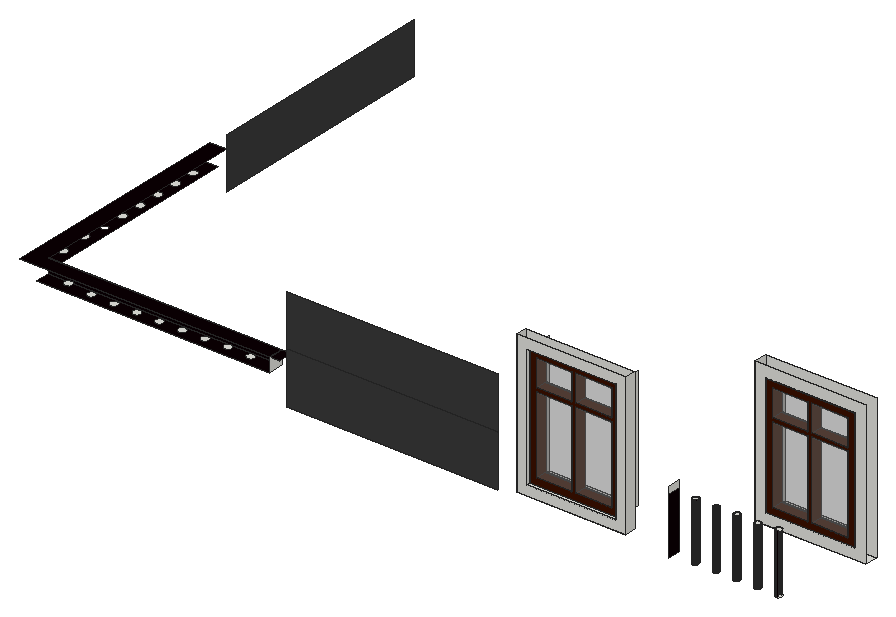
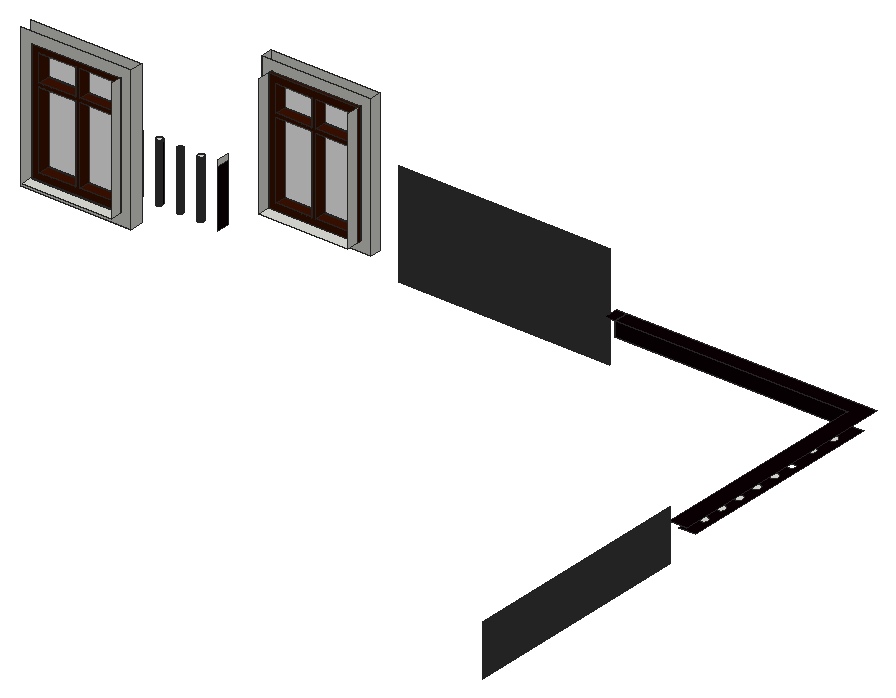
# SketchUp Ruby script. Lengths in inches.
U = 1.inch
M = Sketchup.active_model
def pt(a) = Geom::Point3d.new(a.map { |v| v * U })
def face(e, loops, mat)
  f = e.add_face(loops[0].map { |a| pt(a) })
  loops[1..].each { |l| e.add_face(l.map { |a| pt(a) }).erase! }
  f.material = f.back_material = mat if mat
  f
end
# faces: each face lists its corners as indices into pts; further lists are holes
def faces(e, pts, list, mat = nil) = list.each { |f| face(e, (f[0].is_a?(Array) ? f : [f]).map { |l| l.map { |i| pts[i] } }, mat) }
# xy, xz, yz: faces in a plane at the given z, y or x. An outline is a flat list of corners, or four numbers for a rectangle; further outlines are holes
def ring(l) = l.size == 4 ? [[l[0], l[1]], [l[2], l[1]], [l[2], l[3]], [l[0], l[3]]] : l.each_slice(2).to_a
def flat(e, list, mat, &to3) = list.each { |f| face(e, (f[0].is_a?(Array) ? f : [f]).map { |l| ring(l).map { |u, v| to3.(u, v) } }, mat) }
def xy(e, z, list, mat = nil) = flat(e, list, mat) { |x, y| [x, y, z] }
def xz(e, y, list, mat = nil) = flat(e, list, mat) { |x, z| [x, y, z] }
def yz(e, x, list, mat = nil) = flat(e, list, mat) { |y, z| [x, y, z] }
def lines(e, pts, list) = list.each { |a, b| e.add_line(pt(pts[a]), pt(pts[b])) }
# prism: a flat outline (further loops are holes) pulled along v
def prism(e, loops, v, mat = nil)
  f = face(e, loops, mat); d = Geom::Vector3d.new(v.map { |x| x * U })
  f.pushpull(f.normal.samedirection?(d) ? d.length : -d.length)
end
def box(e, o, s, mat = nil) = prism(e, [[o, [o[0] + s[0], o[1], o[2]], [o[0] + s[0], o[1] + s[1], o[2]], [o[0], o[1] + s[1], o[2]]]], [0, 0, s[2]], mat)
def at(x, y, z, deg = 0) = Geom::Transformation.translation(pt([x, y, z])) * Geom::Transformation.rotation(ORIGIN, Z_AXIS, deg.degrees)
def axes(o, x, y, z) = Geom::Transformation.new([*x, 0, *y, 0, *z, 0, *pt(o).to_a, 1])
def part(name) = M.definitions.add(name)
# library, detail: a bought-in or finely detailed component or shape, given as its bounding box
def library(name, o, s) = part(name).tap { |d| box(d.entities, o, s) }
def detail(e, o, s) = box(e.add_group.entities, o, s)
def put(e, d, t, mat = nil) = e.add_instance(d, t).tap { |i| i.material = mat if mat }
def group(e, t, mat = nil) = e.add_group.tap { |g| g.transformation = t; g.material = mat if mat }.entities
root = M.entities
M.materials.add("[Color C08]").color = [60, 17, 0]
M.materials.add("[Color M07]").color = [58, 58, 58]
M.materials.add("[Metal Seamed]").color = [11, 0, 4]
M.materials.add("[Translucent Glass Gray]").color = [128, 128, 128]
M.materials["[Translucent Glass Gray]"].alpha = 0.5
c1 = part("Group\#3")
xy(c1.entities,0,[[0,0,51.6875,4]],"[Color C08]")
xy(c1.entities,4.05,[[4.05,0,24.41,4],[24.41,0,26.55,4],[26.55,0,47.64,4]],"[Color C08]")
xy(c1.entities,49.59,[[4.05,0,24.41,4],[26.55,0,47.64,4]],"[Color C08]")
xy(c1.entities,51.6875,[[4.05,0,24.41,4],[26.55,0,47.64,4]],"[Color C08]")
xy(c1.entities,67.57,[[4.05,0,24.41,4],[26.55,0,47.64,4]],"[Color C08]")
xy(c1.entities,71.625,[[0,0,51.6875,4]],"[Color C08]")
xz(c1.entities,0,[[[0,0,51.6875,71.625],[4.05,4.05,4.05,49.59,24.41,49.59,24.41,4.05,26.55,4.05,26.55,49.59,47.64,49.59,47.64,4.05],[26.55,51.6875,47.64,67.57],[4.05,51.6875,24.41,67.57]]],"[Color C08]")
xz(c1.entities,0,[[4.05,4.05,24.41,49.59],[26.55,4.05,47.64,49.59],[4.05,51.6875,24.41,67.57],[26.55,51.6875,47.64,67.57]],"[Translucent Glass Gray]")
xz(c1.entities,4,[[[0,0,51.6875,71.625],[4.05,4.05,4.05,49.59,24.41,49.59,24.41,4.05,26.55,4.05,26.55,49.59,47.64,49.59,47.64,4.05],[26.55,51.6875,47.64,67.57],[4.05,51.6875,24.41,67.57]]],"[Color C08]")
yz(c1.entities,0,[[0,0,4,71.625]],"[Color C08]")
yz(c1.entities,4.05,[[0,4.05,4,49.59],[0,51.6875,4,67.57]],"[Color C08]")
yz(c1.entities,24.41,[[0,4.05,4,49.59],[0,51.6875,4,67.57]],"[Color C08]")
yz(c1.entities,26.55,[[0,4.05,4,49.59],[0,51.6875,4,67.57]],"[Color C08]")
yz(c1.entities,47.64,[[0,4.05,4,49.59],[0,51.6875,4,67.57]],"[Color C08]")
yz(c1.entities,51.6875,[[0,0,4,71.625]],"[Color C08]")
xy(root,156,[[381.34,72.62,380.91,72.67,380.5,72.83,380.14,73.09,379.86,73.43,379.6875,73.83,379.62,74.27,379.67,74.71,379.83,75.12,380.09,75.47,380.43,75.75,380.84,75.93,381.27,75.99,381.71,75.94,382.12,75.78,382.48,75.52,382.75,75.18,382.93,74.78,382.99,74.34,382.95,73.9,382.79,73.49,382.53,73.14,382.18,72.86,381.78,72.68],[392.97,72.62,392.53,72.67,392.12,72.83,391.76,73.09,391.49,73.43,391.3125,73.83,391.25,74.27,391.29,74.71,391.45,75.12,391.71,75.47,392.06,75.75,392.46,75.93,392.9,75.99,393.33,75.94,393.75,75.78,394.1,75.52,394.375,75.18,394.55,74.78,394.62,74.34,394.57,73.9,394.41,73.49,394.15,73.14,393.81,72.86,393.4,72.68],[404.59,72.62,404.16,72.67,403.75,72.83,403.39,73.09,403.11,73.43,402.9375,73.83,402.87,74.27,402.92,74.71,403.08,75.12,403.34,75.47,403.68,75.75,404.09,75.93,404.52,75.99,404.96,75.94,405.37,75.78,405.73,75.52,406,75.18,406.18,74.78,406.24,74.34,406.2,73.9,406.04,73.49,405.78,73.14,405.43,72.86,405.03,72.68],[416.22,72.62,415.78,72.67,415.37,72.83,415.01,73.09,414.74,73.43,414.5625,73.83,414.5,74.27,414.54,74.71,414.7,75.12,414.96,75.47,415.31,75.75,415.71,75.93,416.15,75.99,416.58,75.94,417,75.78,417.35,75.52,417.625,75.18,417.8,74.78,417.87,74.34,417.82,73.9,417.66,73.49,417.4,73.14,417.06,72.86,416.65,72.68],[427.84,72.62,427.41,72.67,427,72.83,426.64,73.09,426.36,73.43,426.1875,73.83,426.12,74.27,426.17,74.71,426.33,75.12,426.59,75.47,426.93,75.75,427.34,75.93,427.77,75.99,428.21,75.94,428.62,75.78,428.98,75.52,429.25,75.18,429.43,74.78,429.49,74.34,429.45,73.9,429.29,73.49,429.03,73.14,428.68,72.86,428.28,72.68]])
xy(root,165.94,[[388.97,106.41,451.12,113.66]])
xy(root,166.3,[[291.9,60.85,353.07,67.28]])
xy(root,171.85,[[297.45,60.85,347.52,67.28],[297.45,67.28,347.52,76.28]])
xy(root,171.98,[[395.02,106.41,445.08,113.66],[395.02,113.66,445.08,119.66]])
xy(root,176.54,[[21.75,62.41,152.3,70.73]],"[Metal Seamed]")
xy(root,177,[[61.41,65.07,61.9,65.2,62.34,65.44,62.71,65.79,62.97,66.23,63.11,66.71,63.11,67.22,62.99,67.71,62.75,68.15,62.39,68.52,61.96,68.78,61.47,68.91,60.97,68.92,60.48,68.8,60.03,68.55,59.67,68.2,59.41,67.77,59.27,67.28,59.26,66.78,59.39,66.29,59.63,65.84,59.98,65.48,60.42,65.22,60.9,65.08]])
xy(root,177.0625,[[86.91,65.07,87.4,65.2,87.84,65.44,88.21,65.79,88.47,66.23,88.61,66.71,88.61,67.22,88.49,67.71,88.25,68.15,87.89,68.52,87.46,68.78,86.97,68.91,86.47,68.92,85.98,68.8,85.53,68.55,85.17,68.2,84.91,67.77,84.77,67.28,84.76,66.78,84.89,66.29,85.13,65.84,85.48,65.48,85.92,65.22,86.4,65.08]])
xy(root,177.125,[[74.16,65.07,74.65,65.2,75.09,65.44,75.46,65.79,75.72,66.23,75.86,66.71,75.86,67.22,75.74,67.71,75.5,68.15,75.14,68.52,74.71,68.78,74.22,68.91,73.72,68.92,73.23,68.8,72.78,68.55,72.42,68.2,72.16,67.77,72.02,67.28,72.01,66.78,72.14,66.29,72.38,65.84,72.73,65.48,73.17,65.22,73.65,65.08]])
xy(root,177.1875,[[48.66,65.07,49.15,65.2,49.59,65.44,49.96,65.79,50.22,66.23,50.36,66.71,50.36,67.22,50.24,67.71,50,68.15,49.64,68.52,49.21,68.78,48.72,68.91,48.22,68.92,47.73,68.8,47.28,68.55,46.92,68.2,46.66,67.77,46.52,67.28,46.51,66.78,46.64,66.29,46.88,65.84,47.23,65.48,47.67,65.22,48.15,65.08],[99.66,65.07,100.15,65.2,100.59,65.44,100.96,65.79,101.22,66.23,101.36,66.71,101.36,67.22,101.24,67.71,101,68.15,100.64,68.52,100.21,68.78,99.72,68.91,99.22,68.92,98.73,68.8,98.28,68.55,97.92,68.2,97.66,67.77,97.52,67.28,97.51,66.78,97.64,66.29,97.88,65.84,98.23,65.48,98.67,65.22,99.15,65.08]])
xy(root,177.3125,[[112.41,65.07,112.9,65.2,113.34,65.44,113.71,65.79,113.97,66.23,114.11,66.71,114.11,67.22,113.99,67.71,113.75,68.15,113.39,68.52,112.96,68.78,112.47,68.91,111.97,68.92,111.48,68.8,111.03,68.55,110.67,68.2,110.41,67.77,110.27,67.28,110.26,66.78,110.39,66.29,110.63,65.84,110.98,65.48,111.42,65.22,111.9,65.08]])
xy(root,177.4375,[[137.97,65.07,138.46,65.2,138.91,65.44,139.27,65.79,139.53,66.23,139.67,66.71,139.68,67.22,139.55,67.71,139.31,68.15,138.96,68.52,138.52,68.78,138.04,68.91,137.53,68.92,137.04,68.8,136.6,68.55,136.23,68.2,135.97,67.77,135.83,67.28,135.83,66.78,135.95,66.29,136.2,65.84,136.55,65.48,136.98,65.22,137.47,65.08]])
xy(root,177.75,[[125.16,65.07,125.65,65.2,126.09,65.44,126.46,65.79,126.72,66.23,126.86,66.71,126.86,67.22,126.74,67.71,126.5,68.15,126.14,68.52,125.71,68.78,125.22,68.91,124.72,68.92,124.23,68.8,123.78,68.55,123.42,68.2,123.16,67.77,123.02,67.28,123.01,66.78,123.14,66.29,123.38,65.84,123.73,65.48,124.17,65.22,124.65,65.08]])
xy(root,178.3125,[[35.91,65.07,36.4,65.2,36.84,65.44,37.21,65.79,37.47,66.23,37.61,66.71,37.61,67.22,37.49,67.71,37.25,68.15,36.89,68.52,36.46,68.78,35.97,68.91,35.47,68.92,34.98,68.8,34.53,68.55,34.17,68.2,33.91,67.77,33.77,67.28,33.76,66.78,33.89,66.29,34.13,65.84,34.48,65.48,34.92,65.22,35.4,65.08]])
xy(root,178.35,[[[12.3125,71.24,21.75,188.85],[17.07,113.4,17.62,113.43,18.15,113.6,18.62,113.9,18.99,114.31,19.24,114.8,19.36,115.35,19.33,115.9,19.17,116.43,18.87,116.89,18.45,117.27,17.96,117.52,17.42,117.64,16.87,117.61,16.34,117.44,15.87,117.14,15.5,116.73,15.24,116.24,15.125,115.7,15.15,115.14,15.32,114.62,15.62,114.15,16.03,113.78,16.52,113.52]]],"[Metal Seamed]")
xy(root,178.875,[[17.07,150.34,17.62,150.37,18.15,150.54,18.62,150.84,18.99,151.25,19.24,151.74,19.36,152.28,19.33,152.84,19.17,153.37,18.87,153.83,18.45,154.21,17.96,154.46,17.42,154.58,16.87,154.55,16.34,154.38,15.87,154.08,15.5,153.67,15.24,153.18,15.125,152.64,15.15,152.08,15.32,151.55,15.62,151.09,16.03,150.71,16.52,150.46]])
xy(root,178.9375,[[17.07,138.03,17.62,138.06,18.15,138.22,18.62,138.52,18.99,138.94,19.24,139.43,19.36,139.97,19.33,140.52,19.17,141.05,18.87,141.52,18.45,141.89,17.96,142.15,17.42,142.26,16.87,142.24,16.34,142.07,15.87,141.77,15.5,141.36,15.24,140.87,15.125,140.32,15.15,139.77,15.32,139.24,15.62,138.77,16.03,138.4,16.52,138.15],[17.07,174.97,17.62,174.99,18.15,175.16,18.62,175.46,18.99,175.87,19.24,176.37,19.36,176.91,19.33,177.46,19.17,177.99,18.87,178.46,18.45,178.83,17.96,179.08,17.42,179.2,16.87,179.18,16.34,179.01,15.87,178.71,15.5,178.3,15.24,177.8,15.125,177.26,15.15,176.71,15.32,176.18,15.62,175.71,16.03,175.34,16.52,175.08]])
xy(root,179,[[17.07,125.72,17.62,125.74,18.15,125.91,18.62,126.21,18.99,126.62,19.24,127.12,19.36,127.66,19.33,128.21,19.17,128.74,18.87,129.21,18.45,129.58,17.96,129.83,17.42,129.95,16.87,129.93,16.34,129.76,15.87,129.46,15.5,129.05,15.24,128.55,15.125,128.01,15.15,127.46,15.32,126.93,15.62,126.46,16.03,126.09,16.52,125.83]])
xy(root,179.0625,[[17.07,162.65,17.62,162.68,18.15,162.85,18.62,163.15,18.99,163.56,19.24,164.05,19.36,164.6,19.33,165.15,19.17,165.68,18.87,166.14,18.45,166.52,17.96,166.77,17.42,166.89,16.87,166.86,16.34,166.69,15.87,166.39,15.5,165.98,15.24,165.49,15.125,164.95,15.15,164.39,15.32,163.87,15.62,163.4,16.03,163.03,16.52,162.77]])
xy(root,179.5625,[[17.07,84.28,17.62,84.31,18.15,84.47,18.62,84.77,18.99,85.19,19.24,85.68,19.36,86.22,19.33,86.77,19.17,87.3,18.87,87.77,18.45,88.14,17.96,88.4,17.42,88.51,16.87,88.49,16.34,88.32,15.87,88.02,15.5,87.61,15.24,87.12,15.125,86.57,15.15,86.02,15.32,85.49,15.62,85.02,16.03,84.65,16.52,84.4]])
xy(root,180.25,[[17.07,99.09,17.62,99.12,18.15,99.29,18.62,99.59,18.99,100,19.24,100.49,19.36,101.03,19.33,101.59,19.17,102.12,18.87,102.58,18.45,102.96,17.96,103.21,17.42,103.33,16.87,103.3,16.34,103.13,15.87,102.83,15.5,102.42,15.24,101.93,15.125,101.39,15.15,100.83,15.32,100.3,15.62,99.84,16.03,99.46,16.52,99.21]])
xy(root,184.4375,[[12.3125,62.41,152.3,62.41,152.3,70.73,21.75,70.73,21.75,195.41,12.3125,195.41],[152.3,62.41,158,70.73]],"[Metal Seamed]")
xy(root,188.3125,[[416.22,72.62,416.65,72.68,417.06,72.86,417.4,73.14,417.66,73.49,417.82,73.9,417.87,74.34,417.8,74.78,417.625,75.18,417.35,75.52,417,75.78,416.58,75.94,416.15,75.99,415.71,75.93,415.31,75.75,414.96,75.47,414.7,75.12,414.54,74.71,414.5,74.27,414.5625,73.83,414.74,73.43,415.01,73.09,415.37,72.83,415.78,72.67]])
xy(root,188.4375,[[381.34,72.62,381.78,72.68,382.18,72.86,382.53,73.14,382.79,73.49,382.95,73.9,382.99,74.34,382.93,74.78,382.75,75.18,382.48,75.52,382.12,75.78,381.71,75.94,381.27,75.99,380.84,75.93,380.43,75.75,380.09,75.47,379.83,75.12,379.67,74.71,379.62,74.27,379.6875,73.83,379.86,73.43,380.14,73.09,380.5,72.83,380.91,72.67]])
xy(root,188.75,[[404.59,72.62,405.03,72.68,405.43,72.86,405.78,73.14,406.04,73.49,406.2,73.9,406.24,74.34,406.18,74.78,406,75.18,405.73,75.52,405.37,75.78,404.96,75.94,404.52,75.99,404.09,75.93,403.68,75.75,403.34,75.47,403.08,75.12,402.92,74.71,402.87,74.27,402.9375,73.83,403.11,73.43,403.39,73.09,403.75,72.83,404.16,72.67]])
xy(root,189.4375,[[427.84,72.62,428.28,72.68,428.68,72.86,429.03,73.14,429.29,73.49,429.45,73.9,429.49,74.34,429.43,74.78,429.25,75.18,428.98,75.52,428.62,75.78,428.21,75.94,427.77,75.99,427.34,75.93,426.93,75.75,426.59,75.47,426.33,75.12,426.17,74.71,426.12,74.27,426.1875,73.83,426.36,73.43,426.64,73.09,427,72.83,427.41,72.67]])
xz(root,60.85,[[[291.9,166.3,353.07,245.34],[297.45,171.85,347.52,239.79]]])
xz(root,67.28,[[[291.9,166.3,353.07,245.34],[297.45,171.85,347.52,239.79]]])
xz(root,67.28,[[158,158.9375,275.92,188],[158,188,275.92,217.0625]],"[Color M07]")
xz(root,70.73,[[21.75,176.54,152.3,184.4375]],"[Metal Seamed]")
xz(root,106.41,[[[388.97,165.94,451.12,245.96],[395.02,171.98,445.08,239.92]]])
xz(root,113.66,[[[388.97,165.94,451.12,245.96],[395.02,171.98,445.08,239.92]]])
yz(root,21.75,[[195.41,162.97,326.53,191.53]],"[Color M07]")
yz(root,152.3,[[62.41,176.54,70.73,184.4375]])
yz(root,291.9,[[60.85,166.3,67.28,245.34]])
yz(root,297.45,[[60.85,171.85,67.28,239.79],[67.28,171.85,76.28,239.79]])
yz(root,347.52,[[60.85,171.85,67.28,239.79],[67.28,171.85,76.28,239.79]])
yz(root,353.07,[[60.85,166.3,67.28,245.34]])
yz(root,369.3125,[[70.41,188.2,77.3,192]])
yz(root,369.3125,[[70.41,156,77.3,188.2]],"[Metal Seamed]")
yz(root,388.97,[[106.41,165.94,113.66,245.96]])
yz(root,395.02,[[106.41,171.98,113.66,239.92],[113.66,171.98,119.66,239.92]])
p = [[380.91,72.67,156],[381.34,72.62,156],[381.34,72.62,188.4375],[380.91,72.67,188.4375],[381.78,72.68,156],[381.78,72.68,188.4375],
  [392.53,72.67,156],[392.97,72.62,156],[392.97,72.62,188.2],[392.53,72.67,188.2],[393.4,72.68,156],[393.4,72.68,188.2],
  [404.16,72.67,156],[404.59,72.62,156],[404.59,72.62,188.75],[404.16,72.67,188.75],[405.03,72.68,156],[405.03,72.68,188.75],
  [415.78,72.67,156],[416.22,72.62,156],[416.22,72.62,188.3125],[415.78,72.67,188.3125],[416.65,72.68,156],[416.65,72.68,188.3125],
  [427.41,72.67,156],[427.84,72.62,156],[427.84,72.62,189.4375],[427.41,72.67,189.4375],[428.28,72.68,156],[428.28,72.68,189.4375],
  [380.5,72.83,156],[380.5,72.83,188.4375],[382.18,72.86,156],[382.18,72.86,188.4375],[392.12,72.83,156],[392.12,72.83,188.2],
  [393.81,72.86,156],[393.81,72.86,188.2],[403.75,72.83,156],[403.75,72.83,188.75],[405.43,72.86,156],[405.43,72.86,188.75],
  [415.37,72.83,156],[415.37,72.83,188.3125],[417.06,72.86,156],[417.06,72.86,188.3125],[427,72.83,156],[427,72.83,189.4375],
  [428.68,72.86,156],[428.68,72.86,189.4375],[380.14,73.09,156],[380.14,73.09,188.4375],[391.76,73.09,156],[391.76,73.09,188.2],
  [403.39,73.09,156],[403.39,73.09,188.75],[415.01,73.09,156],[415.01,73.09,188.3125],[426.64,73.09,156],[426.64,73.09,189.4375],
  [382.53,73.14,156],[382.53,73.14,188.4375],[394.15,73.14,156],[394.15,73.14,188.2],[405.78,73.14,156],[405.78,73.14,188.75],
  [417.4,73.14,156],[417.4,73.14,188.3125],[379.86,73.43,156],[379.86,73.43,188.4375],[382.79,73.49,156],[382.79,73.49,188.4375],
  [391.49,73.43,156],[391.49,73.43,188.2],[394.41,73.49,156],[394.41,73.49,188.2],[403.11,73.43,156],[403.11,73.43,188.75],
  [406.04,73.49,156],[406.04,73.49,188.75],[414.74,73.43,156],[414.74,73.43,188.3125],[417.66,73.49,156],[417.66,73.49,188.3125],
  [426.36,73.43,156],[426.36,73.43,189.4375],[379.6875,73.83,156],[379.6875,73.83,188.4375],[391.3125,73.83,156],[391.3125,73.83,188.2],
  [402.9375,73.83,156],[402.9375,73.83,188.75],[414.5625,73.83,156],[414.5625,73.83,188.3125],[426.1875,73.83,156],[426.1875,73.83,189.4375],
  [382.95,73.9,156],[382.95,73.9,188.4375],[394.57,73.9,156],[394.57,73.9,188.2],[406.2,73.9,156],[406.2,73.9,188.75],
  [417.82,73.9,156],[417.82,73.9,188.3125],[379.62,74.27,156],[379.62,74.27,188.4375],[391.25,74.27,156],[391.25,74.27,188.2],
  [402.87,74.27,156],[402.87,74.27,188.75],[414.5,74.27,156],[414.5,74.27,188.3125],[426.12,74.27,156],[426.12,74.27,189.4375],
  [382.99,74.34,156],[382.99,74.34,188.4375],[394.62,74.34,156],[394.62,74.34,188.2],[406.24,74.34,156],[406.24,74.34,188.75],
  [417.87,74.34,156],[417.87,74.34,188.3125],[379.67,74.71,156],[379.67,74.71,188.4375],[382.93,74.78,156],[382.93,74.78,188.4375],
  [391.29,74.71,156],[391.29,74.71,188.2],[394.55,74.78,156],[394.55,74.78,188.2],[402.92,74.71,156],[402.92,74.71,188.75],
  [406.18,74.78,156],[406.18,74.78,188.75],[414.54,74.71,156],[414.54,74.71,188.3125],[417.8,74.78,156],[417.8,74.78,188.3125],
  [426.17,74.71,156],[426.17,74.71,189.4375],[379.83,75.12,156],[379.83,75.12,188.4375],[391.45,75.12,156],[391.45,75.12,188.2],
  [403.08,75.12,156],[403.08,75.12,188.75],[414.7,75.12,156],[414.7,75.12,188.3125],[426.33,75.12,156],[426.33,75.12,189.4375],
  [382.75,75.18,156],[382.75,75.18,188.4375],[394.375,75.18,156],[394.375,75.18,188.2],[406,75.18,156],[406,75.18,188.75],
  [417.625,75.18,156],[417.625,75.18,188.3125],[380.09,75.47,156],[380.09,75.47,188.4375],[391.71,75.47,156],[391.71,75.47,188.2],
  [403.34,75.47,156],[403.34,75.47,188.75],[414.96,75.47,156],[414.96,75.47,188.3125],[426.59,75.47,156],[426.59,75.47,189.4375],
  [382.48,75.52,156],[382.48,75.52,188.4375],[394.1,75.52,156],[394.1,75.52,188.2],[405.73,75.52,156],[405.73,75.52,188.75],
  [417.35,75.52,156],[417.35,75.52,188.3125],[380.43,75.75,156],[380.43,75.75,188.4375],[382.12,75.78,156],[382.12,75.78,188.4375],
  [392.06,75.75,156],[392.06,75.75,188.2],[393.75,75.78,156],[393.75,75.78,188.2],[403.68,75.75,156],[403.68,75.75,188.75],
  [405.37,75.78,156],[405.37,75.78,188.75],[415.31,75.75,156],[415.31,75.75,188.3125],[417,75.78,156],[417,75.78,188.3125],
  [426.93,75.75,156],[426.93,75.75,189.4375],[380.84,75.93,156],[380.84,75.93,188.4375],[392.46,75.93,156],[392.46,75.93,188.2],
  [404.09,75.93,156],[404.09,75.93,188.75],[415.71,75.93,156],[415.71,75.93,188.3125],[427.34,75.93,156],[427.34,75.93,189.4375],
  [381.71,75.94,156],[381.71,75.94,188.4375],[393.33,75.94,156],[393.33,75.94,188.2],[404.96,75.94,156],[404.96,75.94,188.75],
  [416.58,75.94,156],[416.58,75.94,188.3125],[428.62,75.78,156],[428.21,75.94,156],[428.21,75.94,189.4375],[428.62,75.78,189.4375],
  [381.27,75.99,156],[381.27,75.99,188.4375],[392.9,75.99,156],[392.9,75.99,188.2],[404.52,75.99,156],[404.52,75.99,188.75],
  [416.15,75.99,156],[416.15,75.99,188.3125],[427.77,75.99,156],[427.77,75.99,189.4375]]
faces(root,p,[[0,1,2,3],[1,4,5,2],[6,7,8,9],[7,10,11,8],[12,13,14,15],[13,16,17,14],[18,19,20,21],[19,22,23,20],
  [24,25,26,27],[25,28,29,26],[30,0,3,31],[4,32,33,5],[34,6,9,35],[10,36,37,11],[38,12,15,39],[16,40,41,17],
  [42,18,21,43],[22,44,45,23],[46,24,27,47],[28,48,49,29],[50,30,31,51],[52,34,35,53],[54,38,39,55],[56,42,43,57],
  [58,46,47,59],[32,60,61,33],[36,62,63,37],[40,64,65,41],[44,66,67,45],[68,50,51,69],[60,70,71,61],[72,52,53,73],
  [62,74,75,63],[76,54,55,77],[64,78,79,65],[80,56,57,81],[66,82,83,67],[84,58,59,85],[86,68,69,87],[88,72,73,89],
  [90,76,77,91],[92,80,81,93],[94,84,85,95],[70,96,97,71],[74,98,99,75],[78,100,101,79],[82,102,103,83],[104,86,87,105],
  [106,88,89,107],[108,90,91,109],[110,92,93,111],[112,94,95,113],[96,114,115,97],[98,116,117,99],[100,118,119,101],[102,120,121,103],
  [122,104,105,123],[114,124,125,115],[126,106,107,127],[116,128,129,117],[130,108,109,131],[118,132,133,119],[134,110,111,135],[120,136,137,121],
  [138,112,113,139],[140,122,123,141],[142,126,127,143],[144,130,131,145],[146,134,135,147],[148,138,139,149],[124,150,151,125],[128,152,153,129],
  [132,154,155,133],[136,156,157,137],[158,140,141,159],[160,142,143,161],[162,144,145,163],[164,146,147,165],[166,148,149,167],[150,168,169,151],
  [152,170,171,153],[154,172,173,155],[156,174,175,157],[176,158,159,177],[168,178,179,169],[180,160,161,181],[170,182,183,171],[184,162,163,185],
  [172,186,187,173],[188,164,165,189],[174,190,191,175],[192,166,167,193],[194,176,177,195],[196,180,181,197],[198,184,185,199],[200,188,189,201],
  [202,192,193,203],[178,204,205,179],[182,206,207,183],[186,208,209,187],[190,210,211,191],[212,213,214,215],[216,194,195,217],[204,216,217,205],
  [218,196,197,219],[206,218,219,207],[220,198,199,221],[208,220,221,209],[222,200,201,223],[210,222,223,211],[224,202,203,225],[213,224,225,214]],"[Metal Seamed]")
put(root,c1,axes([297.45,62.91,171.85],[0.96856,0,0],[0,1.6104,0],[0,0,0.94852]))
put(root,c1,axes([395.02,106.41,171.98],[0.96856,0,0],[0,1.6104,0],[0,0,0.94852]))
